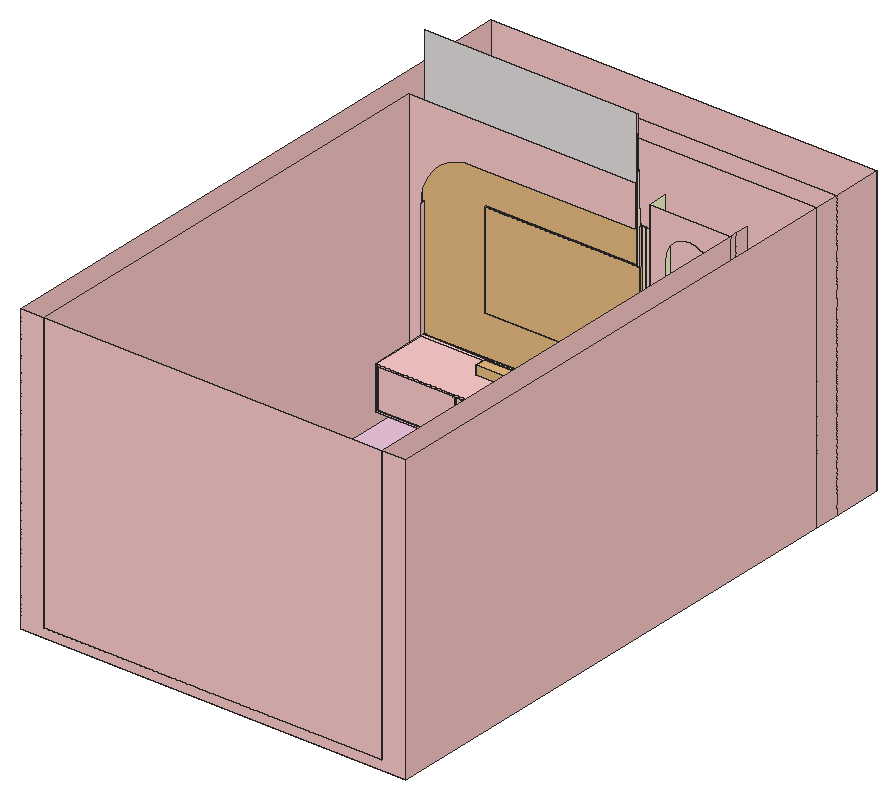
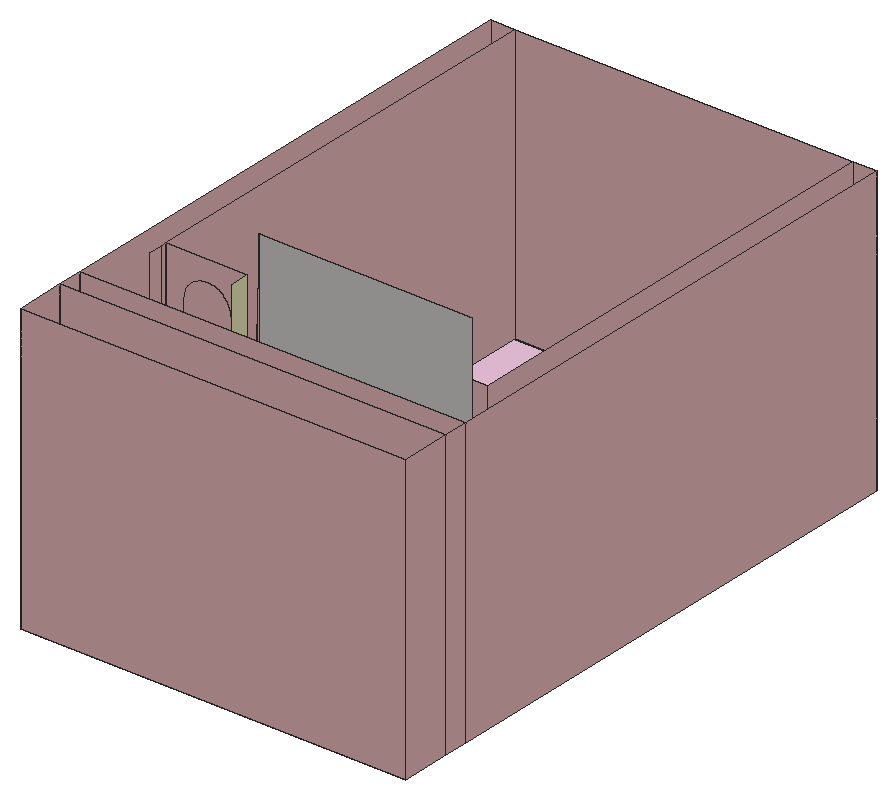
# SketchUp Ruby script. Lengths in inches.
U = 1.inch
M = Sketchup.active_model
def pt(a) = Geom::Point3d.new(a.map { |v| v * U })
def face(e, loops, mat)
  f = e.add_face(loops[0].map { |a| pt(a) })
  loops[1..].each { |l| e.add_face(l.map { |a| pt(a) }).erase! }
  f.material = f.back_material = mat if mat
  f
end
# faces: each face lists its corners as indices into pts; further lists are holes
def faces(e, pts, list, mat = nil) = list.each { |f| face(e, (f[0].is_a?(Array) ? f : [f]).map { |l| l.map { |i| pts[i] } }, mat) }
# xy, xz, yz: faces in a plane at the given z, y or x. An outline is a flat list of corners, or four numbers for a rectangle; further outlines are holes
def ring(l) = l.size == 4 ? [[l[0], l[1]], [l[2], l[1]], [l[2], l[3]], [l[0], l[3]]] : l.each_slice(2).to_a
def flat(e, list, mat, &to3) = list.each { |f| face(e, (f[0].is_a?(Array) ? f : [f]).map { |l| ring(l).map { |u, v| to3.(u, v) } }, mat) }
def xy(e, z, list, mat = nil) = flat(e, list, mat) { |x, y| [x, y, z] }
def xz(e, y, list, mat = nil) = flat(e, list, mat) { |x, z| [x, y, z] }
def yz(e, x, list, mat = nil) = flat(e, list, mat) { |y, z| [x, y, z] }
def lines(e, pts, list) = list.each { |a, b| e.add_line(pt(pts[a]), pt(pts[b])) }
# prism: a flat outline (further loops are holes) pulled along v
def prism(e, loops, v, mat = nil)
  f = face(e, loops, mat); d = Geom::Vector3d.new(v.map { |x| x * U })
  f.pushpull(f.normal.samedirection?(d) ? d.length : -d.length)
end
def box(e, o, s, mat = nil) = prism(e, [[o, [o[0] + s[0], o[1], o[2]], [o[0] + s[0], o[1] + s[1], o[2]], [o[0], o[1] + s[1], o[2]]]], [0, 0, s[2]], mat)
def at(x, y, z, deg = 0) = Geom::Transformation.translation(pt([x, y, z])) * Geom::Transformation.rotation(ORIGIN, Z_AXIS, deg.degrees)
def axes(o, x, y, z) = Geom::Transformation.new([*x, 0, *y, 0, *z, 0, *pt(o).to_a, 1])
def part(name) = M.definitions.add(name)
# library, detail: a bought-in or finely detailed component or shape, given as its bounding box
def library(name, o, s) = part(name).tap { |d| box(d.entities, o, s) }
def detail(e, o, s) = box(e.add_group.entities, o, s)
def put(e, d, t, mat = nil) = e.add_instance(d, t).tap { |i| i.material = mat if mat }
def group(e, t, mat = nil) = e.add_group.tap { |g| g.transformation = t; g.material = mat if mat }.entities
root = M.entities
M.materials.add("Generic").color = [238, 198, 223]
M.materials.add("LIGTH FLOWER DiPTICO I").color = [231, 227, 227]
M.materials.add("[Color A01]").color = [255, 204, 204]
M.materials.add("[Color C01]").color = [255, 229, 204]
M.materials.add("[Color D01]1").color = [255, 242, 204]
M.materials.add("[Color E01]").color = [255, 255, 204]
M.materials.add("[Color M06]").color = [86, 86, 86]
c1 = library("Group\#7",[-0.5,-0.5,-0.1],[134.96,7.57,0.2])
c2 = library("Potted+Plant",[38.42,1.35,0],[44.68,49.99,41.74])
c3 = library("Group\#13",[-0.5,-0.5,0],[93.98,1,74.625])
c4 = library("Group\#20",[-0.5,-0.5,0],[1,1.8125,51.3])
c5 = library("Samsung Speaker Bar",[0,0,0],[55.83,4.44,2.14])
c6 = library("Potted tropical plant",[-29.7,0,-10.87],[31.67,38.52,72.45])
c7 = library("Group\#6",[-0.5,-0.5,0],[21.8125,3.84,10.41])
c8 = library("Group\#5",[-0.5,-0.5,0],[21.8125,3.84,17.08])
c9 = library("Flat panel television",[0,1.41,1.14],[35.92,0.28,20.21])
xy(root,0,[[0,0,166.625,222.04],[0,222.04,166.625,232.97],[0,232.97,166.625,254.47]],"[Color A01]")
xy(root,3.9375,[[10.19,0,156.43,195.09]],"Generic")
xy(root,7.9375,[[15.1,194.59,149.83,195.09],[149.83,194.59,156.43,195.09],[10.19,195.09,15.1,197.47],[15.1,195.09,149.83,197.22],[149.83,195.09,156.43,197.22]],"[Color A01]")
xy(root,13.125,[[15.1,173.22,149.83,188.03],[148.91,188.03,149.0625,194.59,149.83,194.59,149.83,188.03],[149.83,188.72,156.43,191.53],[149.83,191.53,156.43,194.59]],"[Color A01]")
xy(root,13.8125,[[15.1,188.03,15.1,194.59,16.27,188.03]])
xy(root,13.82,[[15.8,173.22,149.14,173.34]],"[Color A01]")
xy(root,14.13,[[16.11,173.22,48.82,173.34],[48.82,173.22,49.13,173.34],[49.69,173.22,82.47,173.34],[82.84,173.22,115.49,173.34],[115.49,173.22,115.8,173.34],
  [116.11,173.22,116.43,173.34],[116.43,173.22,148.82,173.34]],"[Color A01]")
xy(root,30.93,[[16.11,173.22,49.13,173.34],[49.69,173.22,82.16,173.34],[82.16,173.22,82.47,173.34],[82.84,173.22,83.15,173.34],[83.15,173.22,115.8,173.34],
  [116.11,173.22,148.82,173.34]],"[Color A01]")
xy(root,31.24,[[15.8,173.22,82.84,173.34],[82.84,173.22,82.9,173.34],[82.9,173.22,149.14,173.34]],"[Color A01]")
xy(root,31.9375,[[15.1,173.22,149.83,173.22,149.83,188.72,121.1,188.72,121.1,197.22,15.1,197.22],[121.1,188.72,149.83,191.53],[121.1,191.53,149.83,197.22],[15.1,197.22,121.1,197.22,15.1,199.09],[121.1,197.22,121.1,199.66,119.71,199.66,119.71,199.91,119.35,199.91,119.35,199.66,117.96,199.66,117.96,199.91,117.6,199.91,117.6,199.66,116.21,199.66,116.21,199.91,115.85,199.91,115.85,199.66,114.46,199.66,114.46,199.91,114.1,199.91,114.1,199.66,112.71,199.66,112.71,199.91,112.35,199.91,112.35,199.66,110.96,199.66,110.96,199.91,110.6,199.91,110.6,199.66,109.21,199.66,109.21,199.91,108.85,199.91,108.85,199.66,107.54,199.66],
  [14.48,199.09,15.1,199.09,107.46,199.91,14.48,199.91]],"[Color A01]")
xy(root,50.46,[[109.2,198.91,42.01,199.16,42.02,199.91,109.21,199.66]],"[Color A01]")
xz(root,0,[[0,0,166.625,0,166.625,123.9375,156.43,123.9375,156.43,3.9375,10.19,3.9375,10.19,123.9375,0,123.9375],[10.19,3.9375,156.43,123.9375]],"[Color A01]")
xz(root,173.22,[[[15.1,13.125,149.83,31.9375],[15.8,13.82,149.14,31.24]],[16.11,14.13,49.13,30.93],[49.69,14.13,82.47,30.93],[82.84,14.13,115.8,30.93],[116.11,14.13,148.82,30.93]],"[Color A01]")
xz(root,173.34,[[[15.8,13.82,149.14,31.24],[16.11,14.13,49.13,30.93],[82.84,14.13,115.8,30.93],[49.69,14.13,82.47,30.93],[116.11,14.13,148.82,30.93]]],"[Color M06]")
xz(root,188.03,[[15.1,13.125,16.27,13.8125],[16.27,13.125,148.91,13.8125]],"[Color A01]")
xz(root,188.72,[[[149.83,13.125,156.43,13.125,156.43,123.9375,121.1,123.9375,121.1,31.9375,149.83,31.9375],[138.36,33.83,137.82,33.85,137.28,33.89,136.73,33.96,136.2,34.06,135.67,34.1875,135.15,34.34,134.63,34.52,134.13,34.73,133.64,34.97,133.16,35.23,132.7,35.51,132.25,35.82,131.8125,36.15,131.4,36.51,131,36.88,130.63,37.28,130.28,37.69,129.94,38.12,129.64,38.57,129.35,39.04,129.09,39.51,128.86,40.01,128.65,40.51,128.47,41.02,128.3125,41.55,128.18,42.08,128.08,42.61,128.01,43.15,127.97,43.69,127.96,44.24,127.96,104.93,127.97,105.47,128.01,106.01,128.08,106.55,128.18,107.09,128.3125,107.62,128.47,108.14,128.65,108.66,128.86,109.16,129.09,109.65,129.35,110.13,129.64,110.59,129.94,111.04,130.28,111.48,130.63,111.89,131,112.28,131.4,112.66,131.8125,113.01,132.25,113.35,132.7,113.65,133.16,113.9375,133.64,114.2,134.13,114.43,134.63,114.64,135.15,114.82,135.67,114.98,136.2,115.11,136.73,115.2,137.28,115.28,137.82,115.32,138.36,115.33,138.91,115.32,139.45,115.28,139.99,115.2,140.53,115.11,141.06,114.98,141.58,114.82,142.09,114.64,142.6,114.43,143.09,114.2,143.57,113.9375,144.03,113.65,144.48,113.35,144.91,113.01,145.33,112.66,145.72,112.28,146.1,111.89,146.45,111.48,146.78,111.04,147.09,110.59,147.375,110.13,147.63,109.65,147.87,109.16,148.08,108.66,148.26,108.14,148.41,107.62,148.54,107.09,148.64,106.55,148.71,106.01,148.75,105.47,148.77,104.93,148.77,44.24,148.75,43.69,148.71,43.15,148.64,42.61,148.54,42.08,148.41,41.55,148.26,41.02,148.08,40.51,147.87,40.01,147.63,39.51,147.375,39.04,147.09,38.57,146.78,38.12,146.45,37.69,146.1,37.28,145.72,36.88,145.33,36.51,144.91,36.15,144.48,35.82,144.03,35.51,143.57,35.23,143.09,34.97,142.6,34.73,142.09,34.52,141.58,34.34,141.06,34.1875,140.53,34.06,139.99,33.96,139.45,33.89,138.91,33.85]]],"[Color A01]")
xz(root,194.59,[[15.1,7.9375,156.43,7.9375,156.43,13.125,149.0625,13.125,149.0625,13.8125,15.1,13.8125]],"[Color A01]")
xz(root,195.09,[[10.19,3.9375,156.43,7.9375]],"[Color A01]")
xz(root,197.22,[[138.36,33.83,138.91,33.85,139.45,33.89,139.99,33.96,140.53,34.06,141.06,34.1875,141.58,34.34,142.09,34.52,142.6,34.73,143.09,34.97,143.57,35.23,144.03,35.51,144.48,35.82,144.91,36.15,145.33,36.51,145.72,36.88,146.1,37.28,146.45,37.69,146.78,38.12,147.09,38.57,147.375,39.04,147.63,39.51,147.87,40.01,148.08,40.51,148.26,41.02,148.41,41.55,148.54,42.08,148.64,42.61,148.71,43.15,148.75,43.69,148.77,44.24,148.77,61.32,127.96,61.32,127.96,44.24,127.97,43.69,128.01,43.15,128.08,42.61,128.18,42.08,128.3125,41.55,128.47,41.02,128.65,40.51,128.86,40.01,129.09,39.51,129.35,39.04,129.64,38.57,129.94,38.12,130.28,37.69,130.63,37.28,131,36.88,131.4,36.51,131.8125,36.15,132.25,35.82,132.7,35.51,133.16,35.23,133.64,34.97,134.13,34.73,134.63,34.52,135.15,34.34,135.67,34.1875,136.2,34.06,136.73,33.96,137.28,33.89,137.82,33.85]],"[Color A01]")
xz(root,197.47,[[10.19,7.9375,15.1,7.9375,15.1,83.24,15.3,86.2,15.88,89.11,16.83,91.93,18.15,94.59,19.79,97.06,21.75,99.29,23.98,101.25,26.45,102.9,29.12,104.21,31.93,105.16,34.84,105.74,37.8,105.9375,107.98,105.9375,107.98,123.9375,10.19,123.9375]],"[Color A01]")
xz(root,198.91,[[107.54,31.9375,108.85,41.16,108.85,106.5625,107.46,149.43,107.46,32.27]],"[Color C01]")
xz(root,199.09,[[14.48,31.9375,15.1,83.24]],"[Color A01]")
xz(root,199.66,[[15.1,31.36,107.46,149.43],[107.46,31.36,107.54,31.9375,107.46,32.27]],"LIGTH FLOWER DiPTICO I")
xz(root,199.66,[[107.46,31.36,107.46,32.27,107.54,31.9375,108.85,31.9375,108.85,41.16,107.54,31.9375]],"[Color A01]")
xz(root,199.66,[[109.21,31.9375,110.6,106.5625],[110.96,31.9375,112.35,106.5625]],"[Color C01]")
xz(root,199.66,[[116.21,31.9375,117.6,106.5625],[117.96,31.9375,119.35,106.5625]],"[Color D01]1")
xz(root,199.66,[[112.71,31.9375,114.1,106.5625],[114.46,31.9375,115.85,106.5625],[119.71,31.9375,121.1,106.5625]],"[Color E01]")
xz(root,199.91,[[108.85,31.9375,109.21,106.5625],[110.6,31.9375,110.96,106.5625],[112.35,31.9375,112.71,106.5625],[114.1,31.9375,114.46,106.5625],[115.85,31.9375,116.21,106.5625],
  [117.6,31.9375,117.96,106.5625],[119.35,31.9375,119.71,106.5625]],"[Color A01]")
xz(root,209.91,[[138.36,33.83,137.82,33.85,137.28,33.89,136.73,33.96,136.2,34.06,135.67,34.1875,135.15,34.34,134.63,34.52,134.13,34.73,133.64,34.97,133.16,35.23,132.7,35.51,132.25,35.82,131.8125,36.15,131.4,36.51,131,36.88,130.63,37.28,130.28,37.69,129.94,38.12,129.64,38.57,129.35,39.04,129.09,39.51,128.86,40.01,128.65,40.51,128.47,41.02,128.3125,41.55,128.18,42.08,128.08,42.61,128.01,43.15,127.97,43.69,127.96,44.24,127.96,61.32,148.77,61.32,148.77,44.24,148.75,43.69,148.71,43.15,148.64,42.61,148.54,42.08,148.41,41.55,148.26,41.02,148.08,40.51,147.87,40.01,147.63,39.51,147.375,39.04,147.09,38.57,146.78,38.12,146.45,37.69,146.1,37.28,145.72,36.88,145.33,36.51,144.91,36.15,144.48,35.82,144.03,35.51,143.57,35.23,143.09,34.97,142.6,34.73,142.09,34.52,141.58,34.34,141.06,34.1875,140.53,34.06,139.99,33.96,139.45,33.89,138.91,33.85]],"[Color A01]")
xz(root,222.04,[[0,0,166.625,123.9375]],"[Color A01]")
xz(root,232.97,[[0,0,166.625,123.9375]],"[Color A01]")
xz(root,254.47,[[0,0,166.625,123.9375]],"[Color A01]")
yz(root,0,[[0,0,222.04,123.9375],[222.04,0,232.97,123.9375],[232.97,0,254.47,123.9375]],"[Color A01]")
yz(root,10.19,[[0,3.9375,195.09,3.9375,195.09,7.9375,197.47,7.9375,197.47,123.9375,0,123.9375]],"[Color A01]")
yz(root,15.1,[[194.59,7.9375,194.59,13.8125,188.03,13.8125,188.03,13.125,173.22,13.125,173.22,31.9375,197.22,31.9375,197.22,7.9375],[197.22,7.9375,197.47,31.9375],[197.47,31.9375,199.09,83.24]],"[Color A01]")
yz(root,15.8,[[173.22,13.82,173.34,31.24]],"[Color A01]")
yz(root,16.11,[[173.22,14.13,173.34,30.93]],"[Color A01]")
yz(root,49.13,[[173.22,14.13,173.34,30.93]],"[Color A01]")
yz(root,49.69,[[173.22,14.13,173.34,30.93]],"[Color A01]")
yz(root,82.47,[[173.22,14.13,173.34,30.93]],"[Color A01]")
yz(root,82.84,[[173.22,14.13,173.34,30.93]],"[Color A01]")
yz(root,107.46,[[199.91,31.9375,199.66,32.27,199.66,149.43,199.91,106.5625],[198.91,32.27,199.66,149.43]],"[Color A01]")
yz(root,108.85,[[199.66,31.9375,199.91,31.9375,199.91,106.5625,198.91,106.5625,198.91,41.16,199.66,41.16]],"[Color A01]")
yz(root,109.21,[[199.66,31.9375,199.91,106.5625]],"[Color A01]")
yz(root,110.6,[[199.66,31.9375,199.91,106.5625]],"[Color A01]")
yz(root,110.96,[[199.66,31.9375,199.91,106.5625]],"[Color A01]")
yz(root,112.35,[[199.66,31.9375,199.91,106.5625]],"[Color A01]")
yz(root,112.71,[[199.66,31.9375,199.91,106.5625]],"[Color A01]")
yz(root,114.1,[[199.66,31.9375,199.91,106.5625]],"[Color A01]")
yz(root,114.46,[[199.66,31.9375,199.91,106.5625]],"[Color A01]")
yz(root,115.8,[[173.22,14.13,173.34,30.93]],"[Color A01]")
yz(root,115.85,[[199.66,31.9375,199.91,106.5625]],"[Color A01]")
yz(root,116.11,[[173.22,14.13,173.34,30.93]],"[Color A01]")
yz(root,116.21,[[199.66,31.9375,199.91,106.5625]],"[Color A01]")
yz(root,117.6,[[199.66,31.9375,199.91,106.5625]],"[Color A01]")
yz(root,117.96,[[199.66,31.9375,199.91,106.5625]],"[Color A01]")
yz(root,119.35,[[199.66,31.9375,199.91,106.5625]],"[Color A01]")
yz(root,119.71,[[199.66,31.9375,199.91,106.5625]],"[Color A01]")
yz(root,121.1,[[188.72,31.9375,188.72,123.9375,197.22,123.9375,197.22,105.9375,199.09,105.9375,199.09,106.5625,199.66,106.5625,199.66,31.9375]],"[Color E01]")
yz(root,127.96,[[188.72,44.24,194.375,61.32],[197.22,44.24,209.91,61.32]],"[Color A01]")
yz(root,148.77,[[188.72,44.24,194.375,61.32],[197.22,44.24,209.91,61.32]],"[Color A01]")
yz(root,148.82,[[173.22,14.13,173.34,30.93]],"[Color A01]")
yz(root,149.14,[[173.22,13.82,173.34,31.24]],"[Color A01]")
yz(root,149.83,[[173.22,13.125,188.72,31.9375],[188.72,13.125,191.53,31.9375]],"[Color A01]")
yz(root,156.43,[[0,3.9375,0,123.9375,188.72,123.9375,188.72,13.125,194.59,13.125,194.59,7.9375,195.09,7.9375,195.09,3.9375],[194.59,7.9375,194.59,13.125,191.53,13.125,191.53,123.9375,197.22,123.9375,197.22,7.9375],[188.72,13.125,191.53,123.9375]],"[Color A01]")
yz(root,166.625,[[0,0,222.04,123.9375],[222.04,0,232.97,123.9375],[232.97,0,254.47,123.9375]],"[Color A01]")
p = [[16.27,188.03,13.8125],[15.1,194.59,13.8125],[15.1,194.59,13.125],[16.27,188.03,13.125],[149.0625,194.59,13.125],[148.91,188.03,13.125],
  [148.91,188.03,13.8125],[149.0625,194.59,13.8125],[107.46,199.66,32.27],[15.1,199.09,31.9375],[121.1,197.22,31.9375],[107.54,199.66,31.9375],
  [107.54,198.91,31.9375],[107.46,198.91,32.27],[108.85,199.66,41.16],[108.85,198.91,41.16],[107.46,199.91,31.9375],[137.28,194.375,33.89],
  [137.28,188.72,33.89],[137.82,188.72,33.85],[137.82,194.375,33.85],[138.36,188.72,33.83],[138.36,194.375,33.83],[138.91,188.72,33.85],
  [138.91,194.375,33.85],[139.45,188.72,33.89],[139.45,194.375,33.89],[137.82,197.22,33.85],[137.28,197.22,33.89],[137.28,209.91,33.89],
  [137.82,209.91,33.85],[138.36,197.22,33.83],[138.36,209.91,33.83],[138.91,197.22,33.85],[138.91,209.91,33.85],[139.45,197.22,33.89],
  [139.45,209.91,33.89],[136.73,194.375,33.96],[136.73,188.72,33.96],[139.99,188.72,33.96],[139.99,194.375,33.96],[136.73,197.22,33.96],
  [136.73,209.91,33.96],[139.99,197.22,33.96],[139.99,209.91,33.96],[136.2,194.375,34.06],[136.2,188.72,34.06],[140.53,188.72,34.06],
  [140.53,194.375,34.06],[136.2,197.22,34.06],[136.2,209.91,34.06],[140.53,197.22,34.06],[140.53,209.91,34.06],[135.67,194.375,34.1875],
  [135.67,188.72,34.1875],[141.06,188.72,34.1875],[141.06,194.375,34.1875],[135.67,197.22,34.1875],[135.67,209.91,34.1875],[141.06,197.22,34.1875],
  [141.06,209.91,34.1875],[135.15,194.375,34.34],[135.15,188.72,34.34],[141.58,188.72,34.34],[141.58,194.375,34.34],[135.15,197.22,34.34],
  [135.15,209.91,34.34],[141.58,197.22,34.34],[141.58,209.91,34.34],[134.63,194.375,34.52],[134.63,188.72,34.52],[142.09,188.72,34.52],
  [142.09,194.375,34.52],[134.63,197.22,34.52],[134.63,209.91,34.52],[142.09,197.22,34.52],[142.09,209.91,34.52],[134.13,194.375,34.73],
  [134.13,188.72,34.73],[142.6,188.72,34.73],[142.6,194.375,34.73],[134.13,197.22,34.73],[134.13,209.91,34.73],[142.6,197.22,34.73],
  [142.6,209.91,34.73],[133.64,194.375,34.97],[133.64,188.72,34.97],[143.09,188.72,34.97],[143.09,194.375,34.97],[133.64,197.22,34.97],
  [133.64,209.91,34.97],[143.09,197.22,34.97],[143.09,209.91,34.97],[133.16,194.375,35.23],[133.16,188.72,35.23],[143.57,188.72,35.23],
  [143.57,194.375,35.23],[133.16,197.22,35.23],[133.16,209.91,35.23],[143.57,197.22,35.23],[143.57,209.91,35.23],[132.7,194.375,35.51],
  [132.7,188.72,35.51],[144.03,188.72,35.51],[144.03,194.375,35.51],[132.7,197.22,35.51],[132.7,209.91,35.51],[144.03,197.22,35.51],
  [144.03,209.91,35.51],[132.25,194.375,35.82],[132.25,188.72,35.82],[144.48,188.72,35.82],[144.48,194.375,35.82],[132.25,197.22,35.82],
  [132.25,209.91,35.82],[144.48,197.22,35.82],[144.48,209.91,35.82],[131.8125,194.375,36.15],[131.8125,188.72,36.15],[144.91,188.72,36.15],
  [144.91,194.375,36.15],[131.8125,197.22,36.15],[131.8125,209.91,36.15],[144.91,197.22,36.15],[144.91,209.91,36.15],[131.4,194.375,36.51],
  [131.4,188.72,36.51],[145.33,188.72,36.51],[145.33,194.375,36.51],[131.4,197.22,36.51],[131.4,209.91,36.51],[145.33,197.22,36.51],
  [145.33,209.91,36.51],[131,194.375,36.88],[131,188.72,36.88],[145.72,188.72,36.88],[145.72,194.375,36.88],[131,197.22,36.88],
  [131,209.91,36.88],[145.72,197.22,36.88],[145.72,209.91,36.88],[130.63,194.375,37.28],[130.63,188.72,37.28],[146.1,188.72,37.28],
  [146.1,194.375,37.28],[130.63,197.22,37.28],[130.63,209.91,37.28],[146.1,197.22,37.28],[146.1,209.91,37.28],[130.28,194.375,37.69],
  [130.28,188.72,37.69],[146.45,188.72,37.69],[146.45,194.375,37.69],[130.28,197.22,37.69],[130.28,209.91,37.69],[146.45,197.22,37.69],
  [146.45,209.91,37.69],[129.94,194.375,38.12],[129.94,188.72,38.12],[146.78,188.72,38.12],[146.78,194.375,38.12],[129.94,197.22,38.12],
  [129.94,209.91,38.12],[146.78,197.22,38.12],[146.78,209.91,38.12],[129.64,194.375,38.57],[129.64,188.72,38.57],[147.09,188.72,38.57],
  [147.09,194.375,38.57],[129.64,197.22,38.57],[129.64,209.91,38.57],[147.09,197.22,38.57],[147.09,209.91,38.57],[129.35,194.375,39.04],
  [129.35,188.72,39.04],[147.375,188.72,39.04],[147.375,194.375,39.04],[129.35,197.22,39.04],[129.35,209.91,39.04],[147.375,197.22,39.04],
  [147.375,209.91,39.04],[129.09,194.375,39.51],[129.09,188.72,39.51],[147.63,188.72,39.51],[147.63,194.375,39.51],[129.09,197.22,39.51],
  [129.09,209.91,39.51],[147.63,197.22,39.51],[147.63,209.91,39.51],[128.86,194.375,40.01],[128.86,188.72,40.01],[147.87,188.72,40.01],
  [147.87,194.375,40.01],[128.86,197.22,40.01],[128.86,209.91,40.01],[147.87,197.22,40.01],[147.87,209.91,40.01],[128.65,194.375,40.51],
  [128.65,188.72,40.51],[148.08,188.72,40.51],[148.08,194.375,40.51],[128.65,197.22,40.51],[128.65,209.91,40.51],[148.08,197.22,40.51],
  [148.08,209.91,40.51],[128.47,194.375,41.02],[128.47,188.72,41.02],[148.26,188.72,41.02],[148.26,194.375,41.02],[128.47,197.22,41.02],
  [128.47,209.91,41.02],[148.26,197.22,41.02],[148.26,209.91,41.02],[128.3125,194.375,41.55],[128.3125,188.72,41.55],[148.41,188.72,41.55],
  [148.41,194.375,41.55],[128.3125,197.22,41.55],[128.3125,209.91,41.55],[148.41,197.22,41.55],[148.41,209.91,41.55],[128.18,194.375,42.08],
  [128.18,188.72,42.08],[148.54,188.72,42.08],[148.54,194.375,42.08],[128.18,197.22,42.08],[128.18,209.91,42.08],[148.54,197.22,42.08],
  [148.54,209.91,42.08],[128.08,194.375,42.61],[128.08,188.72,42.61],[148.64,188.72,42.61],[148.64,194.375,42.61],[128.08,197.22,42.61],
  [128.08,209.91,42.61],[148.64,197.22,42.61],[148.64,209.91,42.61],[128.01,194.375,43.15],[128.01,188.72,43.15],[148.71,188.72,43.15],
  [148.71,194.375,43.15],[128.01,197.22,43.15],[128.01,209.91,43.15],[148.71,197.22,43.15],[148.71,209.91,43.15],[127.97,194.375,43.69],
  [127.97,188.72,43.69],[148.75,188.72,43.69],[148.75,194.375,43.69],[127.97,197.22,43.69],[127.97,209.91,43.69],[148.75,197.22,43.69],
  [148.75,209.91,43.69],[127.96,194.375,44.24],[127.96,188.72,44.24],[148.77,188.72,44.24],[148.77,194.375,44.24],[127.96,197.22,44.24],
  [127.96,209.91,44.24],[148.77,197.22,44.24],[148.77,209.91,44.24],[109.2,198.91,90.07],[42.01,199.16,90.07],[42.01,199.16,50.46],
  [109.2,198.91,50.46],[109.21,199.66,50.46],[109.21,199.66,90.07],[42.02,199.91,90.07],[42.02,199.91,50.46],[149.83,188.03,13.125],
  [151,188.03,13.125]]
faces(root,p,[[0,1,2,3]])
faces(root,p,[[4,5,6,7],[8,9,10],[11,8,10],[8,11,12,13],[12,11,14,15],[8,16,9],[17,18,19,20],[20,19,21,22],
  [22,21,23,24],[24,23,25,26],[27,28,29,30],[31,27,30,32],[33,31,32,34],[35,33,34,36],[37,38,18,17],[26,25,39,40],
  [28,41,42,29],[43,35,36,44],[45,46,38,37],[40,39,47,48],[41,49,50,42],[51,43,44,52],[53,54,46,45],[48,47,55,56],
  [49,57,58,50],[59,51,52,60],[61,62,54,53],[56,55,63,64],[57,65,66,58],[67,59,60,68],[69,70,62,61],[64,63,71,72],
  [65,73,74,66],[75,67,68,76],[77,78,70,69],[72,71,79,80],[73,81,82,74],[83,75,76,84],[85,86,78,77],[80,79,87,88],
  [81,89,90,82],[91,83,84,92],[93,94,86,85],[88,87,95,96],[89,97,98,90],[99,91,92,100],[101,102,94,93],[96,95,103,104],
  [97,105,106,98],[107,99,100,108],[109,110,102,101],[104,103,111,112],[105,113,114,106],[115,107,108,116],[117,118,110,109],[112,111,119,120],
  [113,121,122,114],[123,115,116,124],[125,126,118,117],[120,119,127,128],[121,129,130,122],[131,123,124,132],[133,134,126,125],[128,127,135,136],
  [129,137,138,130],[139,131,132,140],[141,142,134,133],[136,135,143,144],[137,145,146,138],[147,139,140,148],[149,150,142,141],[144,143,151,152],
  [145,153,154,146],[155,147,148,156],[157,158,150,149],[152,151,159,160],[153,161,162,154],[163,155,156,164],[165,166,158,157],[160,159,167,168],
  [161,169,170,162],[171,163,164,172],[173,174,166,165],[168,167,175,176],[169,177,178,170],[179,171,172,180],[181,182,174,173],[176,175,183,184],
  [177,185,186,178],[187,179,180,188],[189,190,182,181],[184,183,191,192],[185,193,194,186],[195,187,188,196],[197,198,190,189],[192,191,199,200],
  [193,201,202,194],[203,195,196,204],[205,206,198,197],[200,199,207,208],[201,209,210,202],[211,203,204,212],[213,214,206,205],[208,207,215,216],
  [209,217,218,210],[219,211,212,220],[221,222,214,213],[216,215,223,224],[217,225,226,218],[227,219,220,228],[229,230,222,221],[224,223,231,232],
  [225,233,234,226],[235,227,228,236],[237,238,230,229],[232,231,239,240],[233,241,242,234],[243,235,236,244],[245,246,238,237],[240,239,247,248],
  [241,249,250,242],[251,243,244,252],[253,254,246,245],[248,247,255,256],[249,257,258,250],[259,251,252,260],[261,262,263,264],[265,266,261,264],
  [267,268,263,262],[267,266,265,268]],"[Color A01]")
lines(root,p,[[269,270]])
put(root,c1,at(15.1,188.03,13.8125))
put(root,c2,axes([91.22,172.69,31.9375],[0.39,0,0],[0,0.39,0],[0,0,0.39]),"[Color A01]")
put(root,c3,at(14.48,199.91,31.9375),"[Color A01]")
put(root,c4,at(14.48,199.09,31.9375),"[Color A01]")
put(root,c5,axes([46.18,188.37,31.9375],[1.09,0,0],[0,1.09,0],[0,0,1.7004]),"[Color A01]")
put(root,c6,axes([145.91,185.4,37.02],[0.36389,0,0],[0,0.36389,0],[0,0,0.36389]),"[Color A01]")
put(root,c7,at(127.96,194.375,33.83),"[Color A01]")
put(root,c8,at(127.96,194.375,44.24),"[Color A01]")
put(root,c9,axes([42.03,196.02,47.66],[1.8768,0,0],[0,1.8768,0],[0,0,2.02976]),"[Color M06]")
